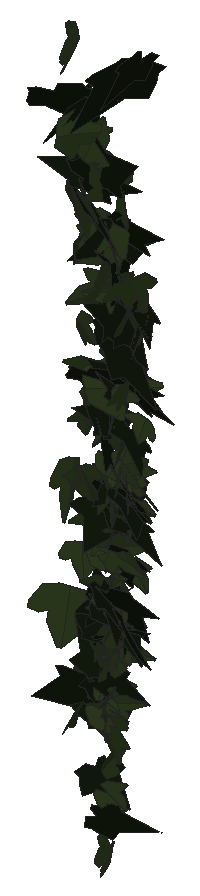
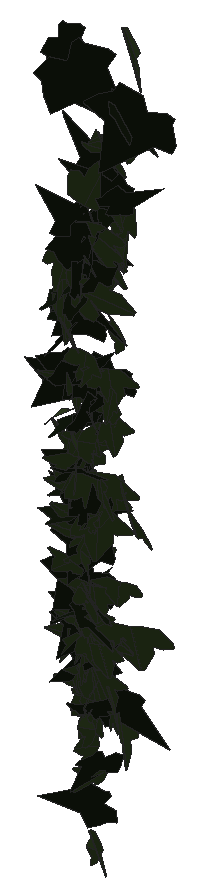
# SketchUp Ruby script. Lengths in inches.
U = 1.inch
M = Sketchup.active_model
def pt(a) = Geom::Point3d.new(a.map { |v| v * U })
def face(e, loops, mat)
  f = e.add_face(loops[0].map { |a| pt(a) })
  loops[1..].each { |l| e.add_face(l.map { |a| pt(a) }).erase! }
  f.material = f.back_material = mat if mat
  f
end
# faces: each face lists its corners as indices into pts; further lists are holes
def faces(e, pts, list, mat = nil) = list.each { |f| face(e, (f[0].is_a?(Array) ? f : [f]).map { |l| l.map { |i| pts[i] } }, mat) }
# xy, xz, yz: faces in a plane at the given z, y or x. An outline is a flat list of corners, or four numbers for a rectangle; further outlines are holes
def ring(l) = l.size == 4 ? [[l[0], l[1]], [l[2], l[1]], [l[2], l[3]], [l[0], l[3]]] : l.each_slice(2).to_a
def flat(e, list, mat, &to3) = list.each { |f| face(e, (f[0].is_a?(Array) ? f : [f]).map { |l| ring(l).map { |u, v| to3.(u, v) } }, mat) }
def xy(e, z, list, mat = nil) = flat(e, list, mat) { |x, y| [x, y, z] }
def xz(e, y, list, mat = nil) = flat(e, list, mat) { |x, z| [x, y, z] }
def yz(e, x, list, mat = nil) = flat(e, list, mat) { |y, z| [x, y, z] }
def lines(e, pts, list) = list.each { |a, b| e.add_line(pt(pts[a]), pt(pts[b])) }
# prism: a flat outline (further loops are holes) pulled along v
def prism(e, loops, v, mat = nil)
  f = face(e, loops, mat); d = Geom::Vector3d.new(v.map { |x| x * U })
  f.pushpull(f.normal.samedirection?(d) ? d.length : -d.length)
end
def box(e, o, s, mat = nil) = prism(e, [[o, [o[0] + s[0], o[1], o[2]], [o[0] + s[0], o[1] + s[1], o[2]], [o[0], o[1] + s[1], o[2]]]], [0, 0, s[2]], mat)
def at(x, y, z, deg = 0) = Geom::Transformation.translation(pt([x, y, z])) * Geom::Transformation.rotation(ORIGIN, Z_AXIS, deg.degrees)
def axes(o, x, y, z) = Geom::Transformation.new([*x, 0, *y, 0, *z, 0, *pt(o).to_a, 1])
def part(name) = M.definitions.add(name)
# library, detail: a bought-in or finely detailed component or shape, given as its bounding box
def library(name, o, s) = part(name).tap { |d| box(d.entities, o, s) }
def detail(e, o, s) = box(e.add_group.entities, o, s)
def put(e, d, t, mat = nil) = e.add_instance(d, t).tap { |i| i.material = mat if mat }
def group(e, t, mat = nil) = e.add_group.tap { |g| g.transformation = t; g.material = mat if mat }.entities
root = M.entities
M.materials.add("1026 AP 7946 SUNNY SIDE UP").color = [254, 231, 186]
M.materials.add("efeu1").color = [18, 25, 13]
M.materials.add("efeu2").color = [43, 57, 29]
c1 = part("ivyleaf_10")
p = [[0,0.5,-0.03],[-0.0625,2.02,-0.43],[-0.19,2.01,-0.46],[-0.54,1.05,-0.29],[-0.52,0.625,-0.18],[-0.83,0.76,-0.28],
  [-1.16,0.64,-0.33],[-1.15,0.33,-0.24],[-0.77,-0.39,0.02],[-0.3,-0.51,0.16],[0.04,-0.48,0.23],[-0.02,2.01,-0.4375],
  [-0.06,2.01,-0.43],[0.04,-0.49,0.23],[0.67,-0.49,0.14],[1.38,0.36,-0.2],[1.375,0.51,-0.24],[0.81,0.65,-0.19],
  [0.62,0.59,-0.15],[0.6,1.09,-0.28],[0.5,1.23,-0.31]]
faces(c1.entities,p,[[0,1,2,3,4,5,6,7,8,9,10],[11,12,0,13,14,15,16,17,18,19,20]],"efeu2")
c2 = part("ivyleaf_9")
p = [[1.54,2.16,1.25],[1.36,2.04,1.19],[-0.21,0.99,0.68],[-0.71,1.11,0.82],[-0.85,0.86,0.67],[-0.8,0.17,0.21],
  [-0.9,-0.01,0.1],[-0.67,-0.16,-0.02],[-0.08,-0.08,-0.05],[-0.03,-0.6,-0.4],[0.65,-0.88,-0.66],[0.83,-0.6,-0.49],
  [1.29,-0.42,-0.43],[1.8125,-0.07,-0.26],[1.21,0.44,0.15]]
faces(c2.entities,p,[[0,1,2,3,4,5,6,7,8,9,10,11,12,13,14]],"efeu1")
put(root,c1,axes([138.35,209.43,255.19],[-0.3379,0.11907,-0.04998],[0.04546,-0.04866,-0.25173],[-0.19741,-0.21502,0.02759]),"1026 AP 7946 SUNNY SIDE UP")
put(root,c1,axes([138.24,209.47,256.97],[0.25643,-0.19179,-0.07868],[0.09738,-0.04594,0.25852],[-0.309,-0.17364,0.01618]),"1026 AP 7946 SUNNY SIDE UP")
put(root,c1,axes([138.08,209.47,256.64],[0.14892,-0.20196,-0.00609],[-0.0155,0.00063,-0.22962],[0.31727,0.09483,-0.00836]),"1026 AP 7946 SUNNY SIDE UP")
put(root,c2,axes([138.12,209.38,254.4375],[0.03624,-0.16423,-0.20982],[-0.03133,0.20182,-0.16957],[0.40905,0.03001,0.0056]),"1026 AP 7946 SUNNY SIDE UP")
put(root,c1,axes([138.31,209.36,254.1],[0.11267,0.15055,0.12818],[0.07966,0.11272,-0.17109],[-0.2957,0.08773,0.00275]),"1026 AP 7946 SUNNY SIDE UP")
put(root,c1,axes([137.71,209.59,261.01],[-0.04402,0.07932,-0.20778],[0.0789,-0.19593,-0.08752],[-0.3322,-0.05705,0.00675]),"1026 AP 7946 SUNNY SIDE UP")
put(root,c2,axes([138.24,209.64,257.46],[0.0235,-0.23346,0.13455],[0.00909,-0.13183,-0.24176],[0.42156,0.01586,-0.00229]),"1026 AP 7946 SUNNY SIDE UP")
put(root,c1,axes([138.28,209.5,258.58],[0.11719,0.00281,0.28805],[0.43919,-0.01413,-0.07664],[0.02033,0.28901,-0.00485]),"1026 AP 7946 SUNNY SIDE UP")
put(root,c2,axes([138.19,209.35,253.58],[0.14345,0.06053,-0.23333],[0.19769,0.19293,0.10626],[0.31176,-0.15019,0.03998]),"1026 AP 7946 SUNNY SIDE UP")
put(root,c2,axes([138.27,209.59,257.17],[0.13961,-0.03347,-0.325],[0.49555,-0.02649,0.09417],[-0.05452,-0.32648,0.02374]),"1026 AP 7946 SUNNY SIDE UP")
put(root,c2,axes([138.13,209.51,257.74],[0.16732,-0.22109,-0.05451],[-0.05164,0.04146,-0.25226],[0.35325,0.11078,-0.01106]),"1026 AP 7946 SUNNY SIDE UP")
put(root,c1,axes([138.32,209.46,255.49],[-0.33073,0.00367,0.06683],[-0.10189,-0.02691,-0.21511],[0.007,-0.21846,0.02632]),"1026 AP 7946 SUNNY SIDE UP")
put(root,c1,axes([138.18,209.61,255.39],[-0.11618,0.11382,0.21675],[0.17248,-0.17881,0.13872],[0.33326,0.13222,0.00377]),"1026 AP 7946 SUNNY SIDE UP")
put(root,c1,axes([137.58,209.4,267.875],[0.18078,-0.30251,-0.18544],[-0.11448,0.16299,-0.33231],[0.54013,0.13579,-0.00837]),"1026 AP 7946 SUNNY SIDE UP")
put(root,c1,axes([138.35,209.45,255.93],[0.05839,-0.20068,-0.06962],[-0.02404,0.06473,-0.20984],[0.33152,0.04004,-0.00296]),"1026 AP 7946 SUNNY SIDE UP")
put(root,c2,axes([138.52,209.47,262.43],[0.21651,-0.28089,-0.15653],[-0.10404,0.135,-0.32148],[0.49004,0.15277,0.00091]),"1026 AP 7946 SUNNY SIDE UP")
put(root,c1,axes([138.36,209.56,257.11],[0.33137,-0.19375,0.04791],[0.03282,-0.04745,-0.29443],[0.31199,0.21078,-0.01991]),"1026 AP 7946 SUNNY SIDE UP")
put(root,c2,axes([138.23,209.36,256.16],[0.01502,-0.03026,-0.2532],[0.09505,0.23863,-0.02647],[0.37733,-0.05891,0.01674]),"1026 AP 7946 SUNNY SIDE UP")
put(root,c1,axes([138.28,209.38,252.68],[0.10972,-0.11384,0.15687],[-0.10111,0.13924,0.13783],[-0.2822,-0.09415,0.01161]),"1026 AP 7946 SUNNY SIDE UP")
put(root,c1,axes([138.27,209.42,252.91],[0.16033,-0.18366,-0.16202],[-0.12126,0.13587,-0.21561],[0.35922,0.12784,-0.00047]),"1026 AP 7946 SUNNY SIDE UP")
put(root,c1,axes([137.61,209.62,262.5],[-0.04785,0.01683,-0.23485],[0.19762,-0.19098,-0.03291],[-0.3004,-0.12832,0.01576]),"1026 AP 7946 SUNNY SIDE UP")
put(root,c1,axes([138.17,209.46,256.62],[-0.29547,0.07792,0.07169],[-0.11354,0.00538,-0.20836],[-0.11808,-0.20015,0.02096]),"1026 AP 7946 SUNNY SIDE UP")
put(root,c1,axes([138.29,209.37,255.36],[0.18572,0.19406,-0.12714],[0.07343,0.11686,0.23396],[0.35504,-0.12568,0.01811]),"1026 AP 7946 SUNNY SIDE UP")
put(root,c1,axes([137.53,209.66,263.96],[-0.00398,-0.11667,-0.21819],[0.018,-0.21096,0.11872],[-0.37887,-0.0088,0.00794]),"1026 AP 7946 SUNNY SIDE UP")
put(root,c2,axes([138.16,209.66,259.16],[-0.30055,-0.19329,0.01803],[0.00032,-0.0263,-0.27955],[0.30534,-0.19023,0.01804]),"1026 AP 7946 SUNNY SIDE UP")
put(root,c2,axes([138.37,209.4,257.77],[0.5301,0.06145,-0.07246],[-0.10018,-0.0431,-0.35189],[-0.10794,0.34175,-0.02925]),"1026 AP 7946 SUNNY SIDE UP")
put(root,c1,axes([138.32,209.53,257.61],[0.36501,0.07574,0.04437],[0.07501,-0.00938,-0.25045],[-0.11424,0.23583,-0.02268]),"1026 AP 7946 SUNNY SIDE UP")
put(root,c1,axes([138.25,209.65,259.4],[0.11803,-0.07072,0.21432],[0.20738,-0.16186,-0.10646],[0.27709,0.15127,-0.01162]),"1026 AP 7946 SUNNY SIDE UP")
put(root,c1,axes([138.29,209.47,256.04],[0.20672,0.17831,0.0706],[0.07355,0.04934,-0.22778],[-0.29064,0.13931,-0.00743]),"1026 AP 7946 SUNNY SIDE UP")
put(root,c2,axes([138.34,209.65,259.81],[0.25931,-0.09997,-0.15621],[0.22739,-0.05038,0.19668],[-0.17154,-0.21789,0.02459]),"1026 AP 7946 SUNNY SIDE UP")
put(root,c2,axes([137.98,209.77,260.5],[0.17283,-0.14142,-0.32274],[0.4215,-0.16929,0.17508],[-0.33645,-0.28472,0.05354]),"1026 AP 7946 SUNNY SIDE UP")
put(root,c1,axes([138.35,209.43,255.72],[-0.08113,-0.0253,0.20894],[0.23693,0.13685,0.05783],[-0.21748,0.15852,-0.01494]),"1026 AP 7946 SUNNY SIDE UP")
put(root,c1,axes([138.34,209.59,258.69],[0.17332,-0.1433,-0.15028],[0.16163,-0.10337,0.18505],[-0.27691,-0.15003,0.01395]),"1026 AP 7946 SUNNY SIDE UP")
put(root,c1,axes([138.43,209.51,256.59],[0.02352,-0.19866,-0.0439],[0.10438,0.0441,-0.19264],[0.30156,0.00023,0.0701]),"1026 AP 7946 SUNNY SIDE UP")
put(root,c1,axes([138.37,209.36,254.57],[0.0437,-0.08544,0.22995],[-0.08449,0.21723,0.09362],[-0.36693,-0.0602,0.00583]),"1026 AP 7946 SUNNY SIDE UP")
put(root,c1,axes([138.42,209.625,256.59],[-0.04497,-0.17946,-0.11573],[-0.04198,-0.10836,0.1864],[-0.3294,0.03831,-0.00795]),"1026 AP 7946 SUNNY SIDE UP")
put(root,c2,axes([137.81,209.54,255.74],[0.02466,0.01918,-0.32053],[-0.4154,-0.16476,-0.02514],[-0.26052,0.26453,0.00974]),"1026 AP 7946 SUNNY SIDE UP")
put(root,c2,axes([137.67,209.62,264.83],[0.24802,-0.23677,0.05639],[0.0283,-0.0553,-0.29298],[0.38155,0.15801,-0.01492]),"1026 AP 7946 SUNNY SIDE UP")
put(root,c2,axes([137.64,209.61,266.72],[-0.3418,0.16986,-0.18457],[0.18554,-0.13965,-0.28318],[-0.34224,-0.24535,0.03082]),"1026 AP 7946 SUNNY SIDE UP")
put(root,c1,axes([138.36,209.5,256.39],[0.26296,-0.1653,0.03653],[-0.02157,0.03777,0.24183],[-0.26527,-0.16693,0.01655]),"1026 AP 7946 SUNNY SIDE UP")
put(root,c1,axes([138.34,209.43,255.85],[0.15389,-0.18439,0.15671],[-0.08074,0.14547,0.21506],[-0.36816,-0.10897,0.01834]),"1026 AP 7946 SUNNY SIDE UP")
put(root,c2,axes([138.53,209.71,259.48],[-0.01762,-0.23264,0.11951],[0.0754,-0.11727,-0.23552],[0.40269,0.01178,0.04933]),"1026 AP 7946 SUNNY SIDE UP")
put(root,c1,axes([138.24,209.65,259.03],[0.15179,-0.13184,0.14149],[0.12617,-0.11239,-0.16899],[0.2724,0.12552,-0.00057]),"1026 AP 7946 SUNNY SIDE UP")
put(root,c2,axes([138.02,209.81,264.13],[0.21508,-0.15685,-0.37707],[0.53982,-0.14786,0.19706],[-0.31473,-0.36079,0.08031]),"1026 AP 7946 SUNNY SIDE UP")
put(root,c1,axes([137.83,209.52,259.43],[-0.30271,0.09561,-0.07098],[-0.08313,0.04902,0.22082],[0.16616,0.1987,-0.01883]),"1026 AP 7946 SUNNY SIDE UP")
put(root,c1,axes([138.22,209.63,255.52],[-0.07532,0.16922,0.14202],[0.06971,-0.12965,0.18033],[0.33508,0.06501,-0.00559]),"1026 AP 7946 SUNNY SIDE UP")
put(root,c1,axes([138.26,209.62,258.74],[0.22808,0.084,-0.12545],[-0.14499,-0.08286,-0.17186],[-0.18268,0.17064,-0.02022]),"1026 AP 7946 SUNNY SIDE UP")
put(root,c1,axes([137.51,209.34,266.15],[-0.01391,-0.03803,-0.3416],[0.31594,0.26398,-0.03519],[0.41863,-0.2005,0.01521]),"1026 AP 7946 SUNNY SIDE UP")
put(root,c2,axes([137.96,209.67,265.47],[-0.01851,0.04565,0.32606],[0.24041,-0.27708,0.04545],[0.44117,0.1529,-0.01108]),"1026 AP 7946 SUNNY SIDE UP")
put(root,c2,axes([138.08,209.55,256.28],[-0.23659,-0.20134,0.10791],[0.07749,0.0951,0.25897],[-0.34922,0.15751,-0.01565]),"1026 AP 7946 SUNNY SIDE UP")
put(root,c2,axes([138.22,209.71,257.35],[0.05596,-0.31772,0.02705],[0.11842,-0.01906,-0.3209],[0.48734,0.04112,0.07487]),"1026 AP 7946 SUNNY SIDE UP")
put(root,c1,axes([138.09,209.59,256.01],[-0.36143,-0.04996,0.11305],[-0.15942,-0.04888,-0.24137],[0.10336,-0.2501,0.02302]),"1026 AP 7946 SUNNY SIDE UP")
put(root,c2,axes([138.23,209.48,256.9375],[-0.35822,0.04481,0.1005],[0.15726,0.007,0.23794],[0.06038,0.24763,-0.02342]),"1026 AP 7946 SUNNY SIDE UP")
put(root,c1,axes([138.72,209.53,263.65],[-0.23461,-0.2606,-0.11785],[0.10817,0.09059,-0.3085],[0.43328,-0.16372,0.0132]),"1026 AP 7946 SUNNY SIDE UP")
put(root,c2,axes([137.85,209.49,261.72],[0.33602,0.13746,-0.04331],[-0.04055,-0.03887,-0.2613],[-0.22273,0.21446,-0.01778]),"1026 AP 7946 SUNNY SIDE UP")
put(root,c1,axes([138.31,209.48,257.12],[0.0269,-0.16167,-0.18068],[-0.02833,0.17353,-0.16646],[0.37293,0.02485,0.00039]),"1026 AP 7946 SUNNY SIDE UP")
put(root,c2,axes([138.26,209.51,258.55],[0.42911,0.05985,-0.10085],[-0.14153,-0.0464,-0.28698],[-0.11264,0.28631,-0.02363]),"1026 AP 7946 SUNNY SIDE UP")
put(root,c1,axes([138.1,209.72,263.25],[-0.15515,-0.30191,-0.12546],[-0.07222,-0.11126,0.32645],[-0.50576,0.1085,-0.00813]),"1026 AP 7946 SUNNY SIDE UP")
put(root,c1,axes([137.55,209.57,264.85],[-0.40891,0.20492,-0.012],[-0.00932,-0.02816,-0.34022],[-0.32271,-0.25885,0.02503]),"1026 AP 7946 SUNNY SIDE UP")
put(root,c1,axes([138.41,209.69,260.125],[0.17495,-0.1091,-0.22113],[0.26968,-0.12909,0.15889],[-0.26451,-0.20378,0.01573]),"1026 AP 7946 SUNNY SIDE UP")
put(root,c1,axes([138.22,209.48,258.55],[-0.09476,-0.05605,0.27655],[0.27327,0.20523,0.08544],[-0.33419,0.18371,-0.00855]),"1026 AP 7946 SUNNY SIDE UP")
put(root,c2,axes([138.21,209.79,260.85],[-0.10875,-0.00591,0.26995],[-0.2843,-0.19518,-0.05483],[0.29846,-0.18808,0.04613]),"1026 AP 7946 SUNNY SIDE UP")
put(root,c1,axes([138.32,209.51,256.92],[-0.10267,-0.0951,0.19636],[0.1412,0.16911,0.11927],[-0.30457,0.11046,-0.0109]),"1026 AP 7946 SUNNY SIDE UP")
put(root,c1,axes([138.08,209.7,255.8],[-0.06493,-0.18025,-0.08915],[0.01131,-0.08862,0.18833],[-0.3135,0.03413,0.02526]),"1026 AP 7946 SUNNY SIDE UP")
put(root,c1,axes([138.24,209.78,263.24],[0.0075,-0.01939,-0.25662],[-0.26329,-0.18502,0.01045],[-0.29136,0.16669,-0.01605]),"1026 AP 7946 SUNNY SIDE UP")
put(root,c1,axes([137.58,209.55,255.34],[0.07153,-0.28961,-0.15725],[-0.04005,0.14885,-0.30114],[0.51201,0.05211,-0.00159]),"1026 AP 7946 SUNNY SIDE UP")
put(root,c1,axes([138.12,209.77,257.69],[-0.04264,0.12324,-0.22786],[0.05832,-0.21882,-0.13116],[-0.3948,-0.04564,0.00524]),"1026 AP 7946 SUNNY SIDE UP")
put(root,c1,axes([138.05,209.75,260.9],[0.09003,-0.02439,0.22203],[0.25844,-0.14079,-0.06218],[0.22288,0.17311,-0.01759]),"1026 AP 7946 SUNNY SIDE UP")
put(root,c1,axes([138.0625,209.55,256.92],[0.00281,0.03962,0.29644],[-0.44892,0.05203,-0.00525],[-0.0822,-0.28279,0.03883]),"1026 AP 7946 SUNNY SIDE UP")
put(root,c1,axes([138.26,209.64,256.41],[0.05306,-0.30235,-0.03139],[0.11054,0.03592,-0.30391],[0.46459,0.02598,0.0759]),"1026 AP 7946 SUNNY SIDE UP")
put(root,c1,axes([137.25,209.69,257.19],[0.55976,0.16102,-0.02231],[-0.01124,-0.03878,-0.40135],[-0.25541,0.35459,-0.03123]),"1026 AP 7946 SUNNY SIDE UP")
put(root,c2,axes([138.47,209.8,260.7],[0.03878,-0.24638,0.08357],[0.04348,-0.07993,-0.25484],[0.40624,0.03208,0.0193]),"1026 AP 7946 SUNNY SIDE UP")
put(root,c2,axes([138.32,209.49,256.95],[0.27813,0.18574,0.05014],[0.07215,0.0219,-0.26347],[-0.29275,0.18186,-0.0173]),"1026 AP 7946 SUNNY SIDE UP")
put(root,c1,axes([137.76,209.69,261.23],[-0.15992,-0.00381,-0.19932],[0.27579,-0.0941,-0.09363],[-0.12847,-0.19726,0.0471]),"1026 AP 7946 SUNNY SIDE UP")
put(root,c2,axes([138.59,209.54,263.02],[-0.21385,-0.0294,-0.36497],[-0.55764,0.03471,0.13756],[0.03459,0.37773,-0.03881]),"1026 AP 7946 SUNNY SIDE UP")
put(root,c2,axes([138.2,209.59,255.34],[-0.37867,-0.05443,0.04752],[0.06351,0.03116,0.2536],[-0.09285,0.24327,-0.02033]),"1026 AP 7946 SUNNY SIDE UP")
put(root,c2,axes([138.66,209.81,267.7],[-0.13635,0.14423,-0.29745],[0.18916,-0.2639,-0.17408],[-0.47217,-0.14737,0.01616]),"1026 AP 7946 SUNNY SIDE UP")
put(root,c1,axes([137.16,209.85,259.5],[0.40035,-0.21318,0.2283],[0.23546,-0.16713,-0.34198],[0.42388,0.29419,-0.02566]),"1026 AP 7946 SUNNY SIDE UP")
put(root,c1,axes([138.31,209.52,257.125],[0.00277,0.12574,-0.19023],[0.00158,0.18537,0.13063],[0.3522,-0.00182,0.00091]),"1026 AP 7946 SUNNY SIDE UP")
put(root,c1,axes([138.06,209.85,263.23],[-0.13354,-0.11038,0.29503],[-0.22638,-0.24883,-0.14393],[0.42725,-0.16635,0.01595]),"1026 AP 7946 SUNNY SIDE UP")
put(root,c1,axes([138.39,209.64,256.71],[0.00706,0.0113,0.21913],[0.31208,0.07685,-0.00807],[-0.12133,0.19832,-0.00802]),"1026 AP 7946 SUNNY SIDE UP")
put(root,c2,axes([138.37,209.77,259.07],[0.12418,-0.26854,0.03029],[0.15966,-0.00039,-0.27061],[0.39393,0.08482,0.10013]),"1026 AP 7946 SUNNY SIDE UP")
put(root,c1,axes([138.26,209.6,259.99],[0.29008,0.07626,-0.11136],[0.1429,0.06274,0.20494],[0.15192,-0.20464,0.01986]),"1026 AP 7946 SUNNY SIDE UP")
put(root,c2,axes([138.4375,209.81,259.9],[0.16369,-0.16372,0.16509],[0.11339,-0.14473,-0.20027],[0.343,0.12598,-0.01258]),"1026 AP 7946 SUNNY SIDE UP")
put(root,c1,axes([138.16,209.81,258.4],[0.03879,-0.13328,0.15504],[0.08789,-0.14188,-0.13902],[0.30456,0.05792,0.02038]),"1026 AP 7946 SUNNY SIDE UP")
put(root,c1,axes([138.12,209.57,259.61],[0.12613,-0.15189,-0.2451],[-0.21625,0.19394,-0.17482],[0.38629,0.15817,-0.01784]),"1026 AP 7946 SUNNY SIDE UP")
put(root,c1,axes([137.76,209.7,261.75],[-0.32601,-0.11413,0.04218],[-0.0414,-0.0381,-0.24313],[0.18646,-0.208,0.01976]),"1026 AP 7946 SUNNY SIDE UP")
put(root,c1,axes([138.36,209.8,260.49],[0.11724,-0.15798,0.12519],[0.06803,-0.1148,-0.18045],[0.3068,0.08583,-0.00783]),"1026 AP 7946 SUNNY SIDE UP")
put(root,c1,axes([137.7,209.7,260.83],[-0.12769,-0.20648,-0.00204],[0.01205,-0.00215,-0.22844],[0.32444,-0.08118,0.00768]),"1026 AP 7946 SUNNY SIDE UP")
put(root,c1,axes([138.25,209.85,264.96],[0.09775,-0.06075,0.26156],[0.2968,-0.17035,-0.09048],[0.28433,0.1987,0.00453]),"1026 AP 7946 SUNNY SIDE UP")
put(root,c1,axes([138.45,209.79,259.79],[-0.03882,0.19859,-0.15783],[0.03,-0.15315,-0.20706],[-0.39434,-0.0312,-0.00021]),"1026 AP 7946 SUNNY SIDE UP")
put(root,c1,axes([138.45,209.71,261.55],[0.00909,-0.28975,-0.0271],[0.04342,0.0251,-0.29702],[0.45519,0.00339,0.02887]),"1026 AP 7946 SUNNY SIDE UP")
put(root,c2,axes([137.6,209.74,265.15],[0.1172,-0.01665,0.27359],[0.34054,-0.15661,-0.07363],[0.24335,0.22717,-0.02874]),"1026 AP 7946 SUNNY SIDE UP")
put(root,c1,axes([138.43,209.73,259.55],[-0.13382,0.00924,-0.20802],[0.29893,-0.07092,-0.08628],[-0.1082,-0.20738,0.01889]),"1026 AP 7946 SUNNY SIDE UP")
put(root,c1,axes([138.21,209.79,263.9],[0.25631,-0.19022,0.06807],[0.04831,-0.06193,-0.25788],[0.3135,0.16506,-0.01591]),"1026 AP 7946 SUNNY SIDE UP")
put(root,c2,axes([138.21,209.63,259.58],[0.38412,0.05699,-0.12345],[-0.17499,-0.04997,-0.2578],[-0.11448,0.26761,-0.02015]),"1026 AP 7946 SUNNY SIDE UP")
put(root,c2,axes([138.4375,209.84,259.82],[-0.35412,-0.09824,0.0222],[-0.0155,-0.0324,-0.25193],[0.15758,-0.22396,0.02511]),"1026 AP 7946 SUNNY SIDE UP")
put(root,c1,axes([137.98,209.71,259.01],[-0.30695,-0.2427,-0.0224],[0.04367,0.00374,-0.32023],[0.38046,-0.19623,0.01869]),"1026 AP 7946 SUNNY SIDE UP")
put(root,c1,axes([138.17,209.61,258.23],[0.25022,0.20004,-0.08353],[0.06047,0.07427,0.26329],[0.33465,-0.16299,0.01488]),"1026 AP 7946 SUNNY SIDE UP")
put(root,c2,axes([137.17,209.52,266.72],[0.49175,0.23747,0.00623],[0.03321,-0.02007,-0.40357],[-0.37199,0.31213,-0.0278]),"1026 AP 7946 SUNNY SIDE UP")
put(root,c2,axes([138.4,209.88,267.38],[-0.10076,0.24731,-0.40049],[0.12036,-0.38276,-0.26514],[-0.7163,-0.0991,0.01178]),"1026 AP 7946 SUNNY SIDE UP")
put(root,c1,axes([138.03,209.89,265.1],[-0.19314,-0.23915,-0.20793],[-0.16942,-0.1697,0.27556],[-0.46051,0.16273,-0.01417]),"1026 AP 7946 SUNNY SIDE UP")
put(root,c2,axes([138.48,209.84,261.4375],[0.18945,-0.12771,0.22003],[0.20756,-0.16931,-0.18139],[0.33286,0.17826,-0.01212]),"1026 AP 7946 SUNNY SIDE UP")
put(root,c1,axes([138.3125,209.59,259.65],[-0.02765,0.1476,0.16764],[-0.03196,0.16061,-0.15219],[-0.34299,-0.02686,0.00067]),"1026 AP 7946 SUNNY SIDE UP")
put(root,c1,axes([138.03,209.57,261.48],[0.17711,-0.06883,-0.35659],[0.50708,0.16676,0.07501],[0.22394,-0.32315,0.11218]),"1026 AP 7946 SUNNY SIDE UP")
put(root,c2,axes([137.82,209.88,263.6],[0.37501,-0.14087,-0.08619],[0.13195,-0.02025,0.28415],[-0.22053,-0.25167,0.02344]),"1026 AP 7946 SUNNY SIDE UP")
put(root,c1,axes([137.96,209.75,259.73],[-0.43229,-0.21229,0.01491],[0.00665,-0.03105,-0.35693],[0.33465,-0.27362,0.02635]),"1026 AP 7946 SUNNY SIDE UP")
put(root,c2,axes([138.1875,209.92,263.33],[0.04159,0.10176,0.34605],[-0.18482,-0.31423,0.10595],[0.5191,-0.12003,0.00999]),"1026 AP 7946 SUNNY SIDE UP")
put(root,c1,axes([137.83,209.55,255.64],[-0.01156,0.05459,0.31429],[-0.35401,0.20834,-0.04282],[-0.33421,-0.22257,0.03448]),"1026 AP 7946 SUNNY SIDE UP")
put(root,c2,axes([138.25,209.75,262.65],[-0.10905,-0.11331,-0.21011],[0.23734,0.1396,-0.13238],[0.2786,-0.16327,0.03053]),"1026 AP 7946 SUNNY SIDE UP")
put(root,c1,axes([138.22,209.59,255.05],[0.11094,-0.12265,0.2205],[-0.13077,0.19852,0.14613],[-0.36618,-0.10806,0.01462]),"1026 AP 7946 SUNNY SIDE UP")
put(root,c1,axes([137.7,209.71,265.71],[0.44077,-0.12665,-0.02671],[0.05653,0.01867,0.31531],[-0.19503,-0.28082,0.03103]),"1026 AP 7946 SUNNY SIDE UP")
put(root,c2,axes([138.4375,209.86,261.48],[0.0231,0.05516,0.26768],[-0.37749,-0.10788,0.03699],[0.1776,-0.23649,0.04382]),"1026 AP 7946 SUNNY SIDE UP")
put(root,c1,axes([138.03,209.79,264.39],[0.44713,-0.09544,-0.15531],[-0.24018,0.01445,-0.30724],[0.14363,0.32127,-0.03027]),"1026 AP 7946 SUNNY SIDE UP")
put(root,c2,axes([138.0625,209.57,257.34],[-0.33883,0.10912,-0.17344],[-0.21802,0.09882,0.24848],[0.22914,0.25539,-0.02005]),"1026 AP 7946 SUNNY SIDE UP")
put(root,c2,axes([138.06,209.92,259.27],[0.11854,-0.10359,0.28039],[0.20601,-0.2397,-0.13249],[0.40993,0.15042,-0.0145]),"1026 AP 7946 SUNNY SIDE UP")
put(root,c1,axes([138.01,209.78,264.12],[0.41627,-0.1412,-0.16112],[-0.24002,0.04274,-0.30727],[0.22703,0.30408,-0.02943]),"1026 AP 7946 SUNNY SIDE UP")
put(root,c1,axes([138.56,209.92,262.68],[0.35924,-0.29674,0.14481],[0.10485,-0.12783,-0.3858],[0.50671,0.23684,-0.02283]),"1026 AP 7946 SUNNY SIDE UP")
put(root,c2,axes([138.51,209.94,263.11],[0.04144,-0.26008,0.10091],[0.04706,-0.09665,-0.26918],[0.43528,0.03521,0.01949]),"1026 AP 7946 SUNNY SIDE UP")
put(root,c1,axes([138,209.79,257.7],[-0.2966,-0.12272,0.02851],[-0.02163,-0.03072,-0.23126],[0.19688,-0.18826,0.01755]),"1026 AP 7946 SUNNY SIDE UP")
put(root,c2,axes([138.2,209.67,260.78],[-0.1953,-0.15579,0.24422],[0.21765,0.19371,0.20622],[-0.39067,0.1858,-0.0072]),"1026 AP 7946 SUNNY SIDE UP")
put(root,c1,axes([138.02,209.81,256.82],[-0.21282,-0.16248,0.03384],[-0.0178,-0.03444,-0.21764],[0.26034,-0.13518,0.01278]),"1026 AP 7946 SUNNY SIDE UP")
put(root,c2,axes([138.26,209.83,264.42],[0.33071,-0.01735,-0.16455],[0.25099,0.05115,0.21123],[0.02741,-0.25904,0.05115]),"1026 AP 7946 SUNNY SIDE UP")
put(root,c1,axes([137.97,209.85,257.23],[-0.11059,-0.1869,0.07351],[-0.0352,-0.06894,-0.2061],[0.3132,-0.07374,0.00279]),"1026 AP 7946 SUNNY SIDE UP")
put(root,c1,axes([137.92,209.79,259.13],[0.05603,0.19841,-0.03395],[-0.00375,-0.0342,-0.20783],[-0.31652,0.03552,-0.00355]),"1026 AP 7946 SUNNY SIDE UP")
put(root,c2,axes([138.43,209.96,262.86],[0.2857,-0.2553,-0.02768],[0.05171,-0.00771,0.32196],[-0.40009,-0.1833,0.02185]),"1026 AP 7946 SUNNY SIDE UP")
put(root,c1,axes([138.41,209.75,259.98],[0.25508,0.1798,0.09318],[0.11194,0.056,-0.24871],[-0.29525,0.17657,-0.0138]),"1026 AP 7946 SUNNY SIDE UP")
put(root,c1,axes([138.58,209.79,263.03],[0.0644,-0.3789,-0.07037],[0.06374,0.07041,-0.38919],[0.60143,0.03311,0.04878]),"1026 AP 7946 SUNNY SIDE UP")
put(root,c1,axes([138.3,209.84,259.89],[0.12871,-0.27764,0.03725],[0.16572,-0.00592,-0.28041],[0.40823,0.08994,0.10209]),"1026 AP 7946 SUNNY SIDE UP")
put(root,c2,axes([138.18,209.8,257.41],[-0.16943,0.20019,-0.09167],[0.0478,-0.08582,-0.23434],[-0.34188,-0.11121,0.01267]),"1026 AP 7946 SUNNY SIDE UP")
put(root,c2,axes([138.37,209.7,261.6],[0.44908,0.07049,0.01676],[0.03409,-0.02189,-0.30196],[-0.10838,0.2852,-0.02554]),"1026 AP 7946 SUNNY SIDE UP")
put(root,c1,axes([138.18,209.8,260.51],[-0.29937,-0.00392,-0.07402],[0.1125,-0.03142,-0.19379],[-0.01175,-0.20105,0.03052]),"1026 AP 7946 SUNNY SIDE UP")
put(root,c1,axes([137.6875,209.77,261.45],[-0.26943,0.14101,0.0334],[-0.0553,0.00688,-0.22791],[-0.22039,-0.17411,0.01636]),"1026 AP 7946 SUNNY SIDE UP")
put(root,c1,axes([138.32,209.75,258.92],[-0.09886,-0.12551,0.14966],[0.16287,0.1074,0.14171],[-0.25517,0.11717,0.03247]),"1026 AP 7946 SUNNY SIDE UP")
put(root,c1,axes([138.63,209.96,260.83],[-0.19442,-0.07033,0.15129],[0.13795,-0.18443,-0.01593],[0.21636,0.0544,0.14611]),"1026 AP 7946 SUNNY SIDE UP")
put(root,c1,axes([137.73,209.62,264.76],[0.01511,0.0235,-0.30324],[-0.18912,0.26943,0.01968],[0.42429,0.11926,0.01957]),"1026 AP 7946 SUNNY SIDE UP")
put(root,c2,axes([138.25,209.99,264.28],[-0.03014,0.02841,-0.32393],[-0.03602,-0.31447,-0.02965],[-0.49538,0.02114,0.02187]),"1026 AP 7946 SUNNY SIDE UP")
put(root,c1,axes([138.43,209.7,256.66],[-0.01853,0.15103,0.13914],[-0.0174,0.13375,-0.15528],[-0.31722,-0.01616,0.00039]),"1026 AP 7946 SUNNY SIDE UP")
put(root,c1,axes([138.1875,209.81,261.98],[-0.35057,0.07121,0.01169],[-0.02827,-0.02054,-0.23985],[-0.1097,-0.22227,0.02447]),"1026 AP 7946 SUNNY SIDE UP")
put(root,c1,axes([137.98,210.02,260.59],[0.00043,-0.10461,0.24559],[0.05,-0.23719,-0.10839],[0.40714,0.02924,0.01305]),"1026 AP 7946 SUNNY SIDE UP")
put(root,c1,axes([138.45,209.85,258.15],[0.238,0.02804,0.13708],[0.21171,-0.00472,-0.15697],[-0.02818,0.20137,-0.02156]),"1026 AP 7946 SUNNY SIDE UP")
put(root,c1,axes([137.41,209.85,258.09],[0.33795,0.08844,0.02717],[0.04958,-0.00889,-0.23858],[-0.13615,0.21629,-0.01944]),"1026 AP 7946 SUNNY SIDE UP")
put(root,c1,axes([137.83,209.8,256.72],[0.30013,0.05156,-0.04684],[-0.0955,0.06206,-0.1886],[-0.05127,0.18621,0.07712]),"1026 AP 7946 SUNNY SIDE UP")
put(root,c2,axes([137.47,209.97,265.125],[-0.07746,-0.00183,0.25347],[-0.3455,-0.11262,-0.04685],[0.17415,-0.22425,0.01981]),"1026 AP 7946 SUNNY SIDE UP")
put(root,c1,axes([138.07,209.81,257.52],[0.29262,-0.08744,0.01092],[-0.00361,0.02111,0.21113],[-0.13855,-0.18523,0.01757]),"1026 AP 7946 SUNNY SIDE UP")
